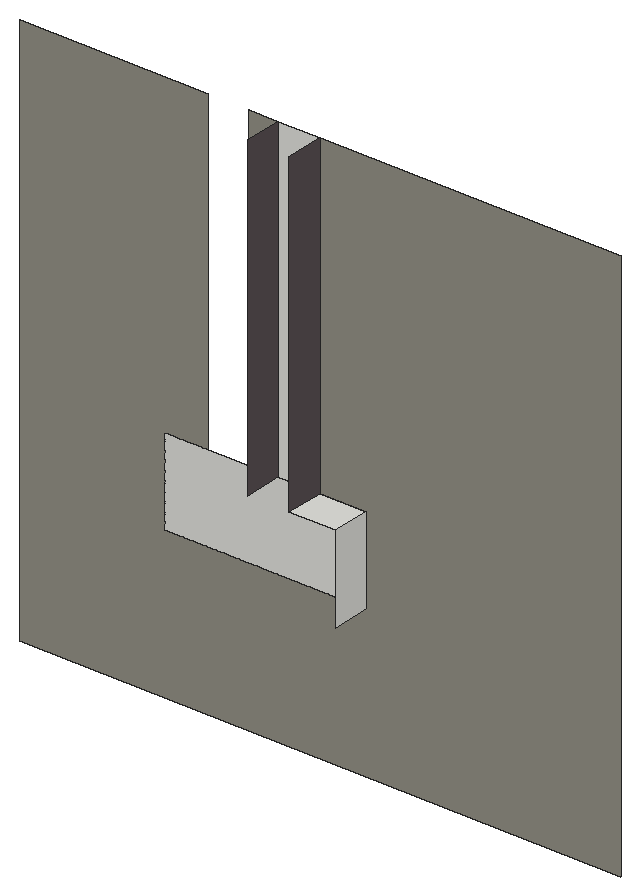
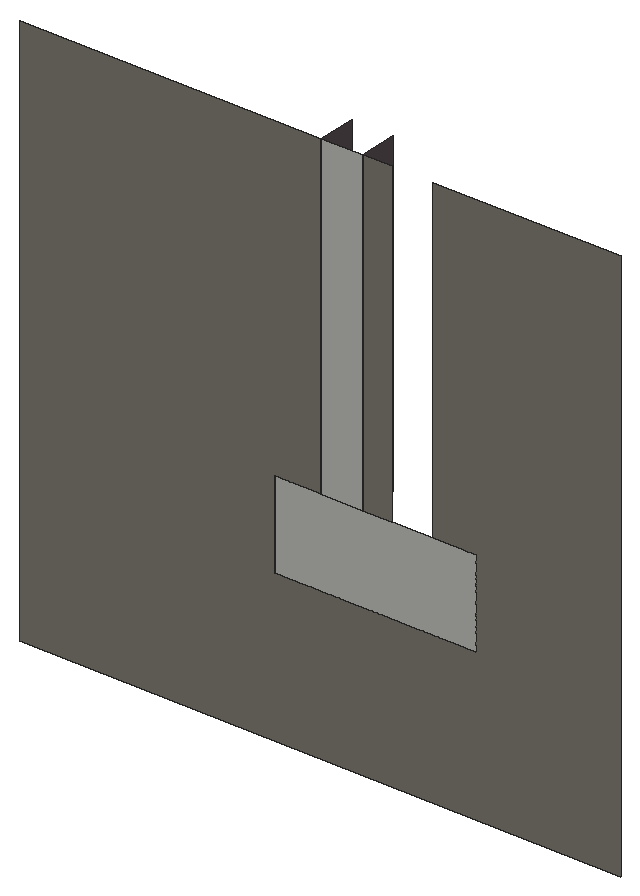
# SketchUp Ruby script. Lengths in inches.
U = 1.inch
M = Sketchup.active_model
def pt(a) = Geom::Point3d.new(a.map { |v| v * U })
def face(e, loops, mat)
  f = e.add_face(loops[0].map { |a| pt(a) })
  loops[1..].each { |l| e.add_face(l.map { |a| pt(a) }).erase! }
  f.material = f.back_material = mat if mat
  f
end
# faces: each face lists its corners as indices into pts; further lists are holes
def faces(e, pts, list, mat = nil) = list.each { |f| face(e, (f[0].is_a?(Array) ? f : [f]).map { |l| l.map { |i| pts[i] } }, mat) }
# xy, xz, yz: faces in a plane at the given z, y or x. An outline is a flat list of corners, or four numbers for a rectangle; further outlines are holes
def ring(l) = l.size == 4 ? [[l[0], l[1]], [l[2], l[1]], [l[2], l[3]], [l[0], l[3]]] : l.each_slice(2).to_a
def flat(e, list, mat, &to3) = list.each { |f| face(e, (f[0].is_a?(Array) ? f : [f]).map { |l| ring(l).map { |u, v| to3.(u, v) } }, mat) }
def xy(e, z, list, mat = nil) = flat(e, list, mat) { |x, y| [x, y, z] }
def xz(e, y, list, mat = nil) = flat(e, list, mat) { |x, z| [x, y, z] }
def yz(e, x, list, mat = nil) = flat(e, list, mat) { |y, z| [x, y, z] }
def lines(e, pts, list) = list.each { |a, b| e.add_line(pt(pts[a]), pt(pts[b])) }
# prism: a flat outline (further loops are holes) pulled along v
def prism(e, loops, v, mat = nil)
  f = face(e, loops, mat); d = Geom::Vector3d.new(v.map { |x| x * U })
  f.pushpull(f.normal.samedirection?(d) ? d.length : -d.length)
end
def box(e, o, s, mat = nil) = prism(e, [[o, [o[0] + s[0], o[1], o[2]], [o[0] + s[0], o[1] + s[1], o[2]], [o[0], o[1] + s[1], o[2]]]], [0, 0, s[2]], mat)
def at(x, y, z, deg = 0) = Geom::Transformation.translation(pt([x, y, z])) * Geom::Transformation.rotation(ORIGIN, Z_AXIS, deg.degrees)
def axes(o, x, y, z) = Geom::Transformation.new([*x, 0, *y, 0, *z, 0, *pt(o).to_a, 1])
def part(name) = M.definitions.add(name)
# library, detail: a bought-in or finely detailed component or shape, given as its bounding box
def library(name, o, s) = part(name).tap { |d| box(d.entities, o, s) }
def detail(e, o, s) = box(e.add_group.entities, o, s)
def put(e, d, t, mat = nil) = e.add_instance(d, t).tap { |i| i.material = mat if mat }
def group(e, t, mat = nil) = e.add_group.tap { |g| g.transformation = t; g.material = mat if mat }.entities
root = M.entities
M.materials.add("[Asphalt New]").color = [91, 82, 84]
M.materials.add("[Formica Graystone]").color = [149, 146, 135]
xy(root,24.68,[[346.48,92.3,351.27,96.24]])
xz(root,96.24,[[330.33,15.61,351.27,24.68],[342.12,24.68,346.48,57.8125]])
xz(root,96.24,[[315.3,0,377.8125,0,377.8125,57.8125,346.48,57.8125,346.48,24.68,351.27,24.68,351.27,15.61,330.33,15.61,330.33,24.68,334.81,24.68,334.81,57.8125,315.3,57.8125],[339.17,24.68,342.12,57.8125]],"[Formica Graystone]")
yz(root,342.12,[[92.3,24.68,96.24,57.8125]],"[Asphalt New]")
yz(root,346.48,[[92.3,24.68,96.24,57.8125]],"[Asphalt New]")
yz(root,351.27,[[92.3,15.61,96.24,24.68]])
